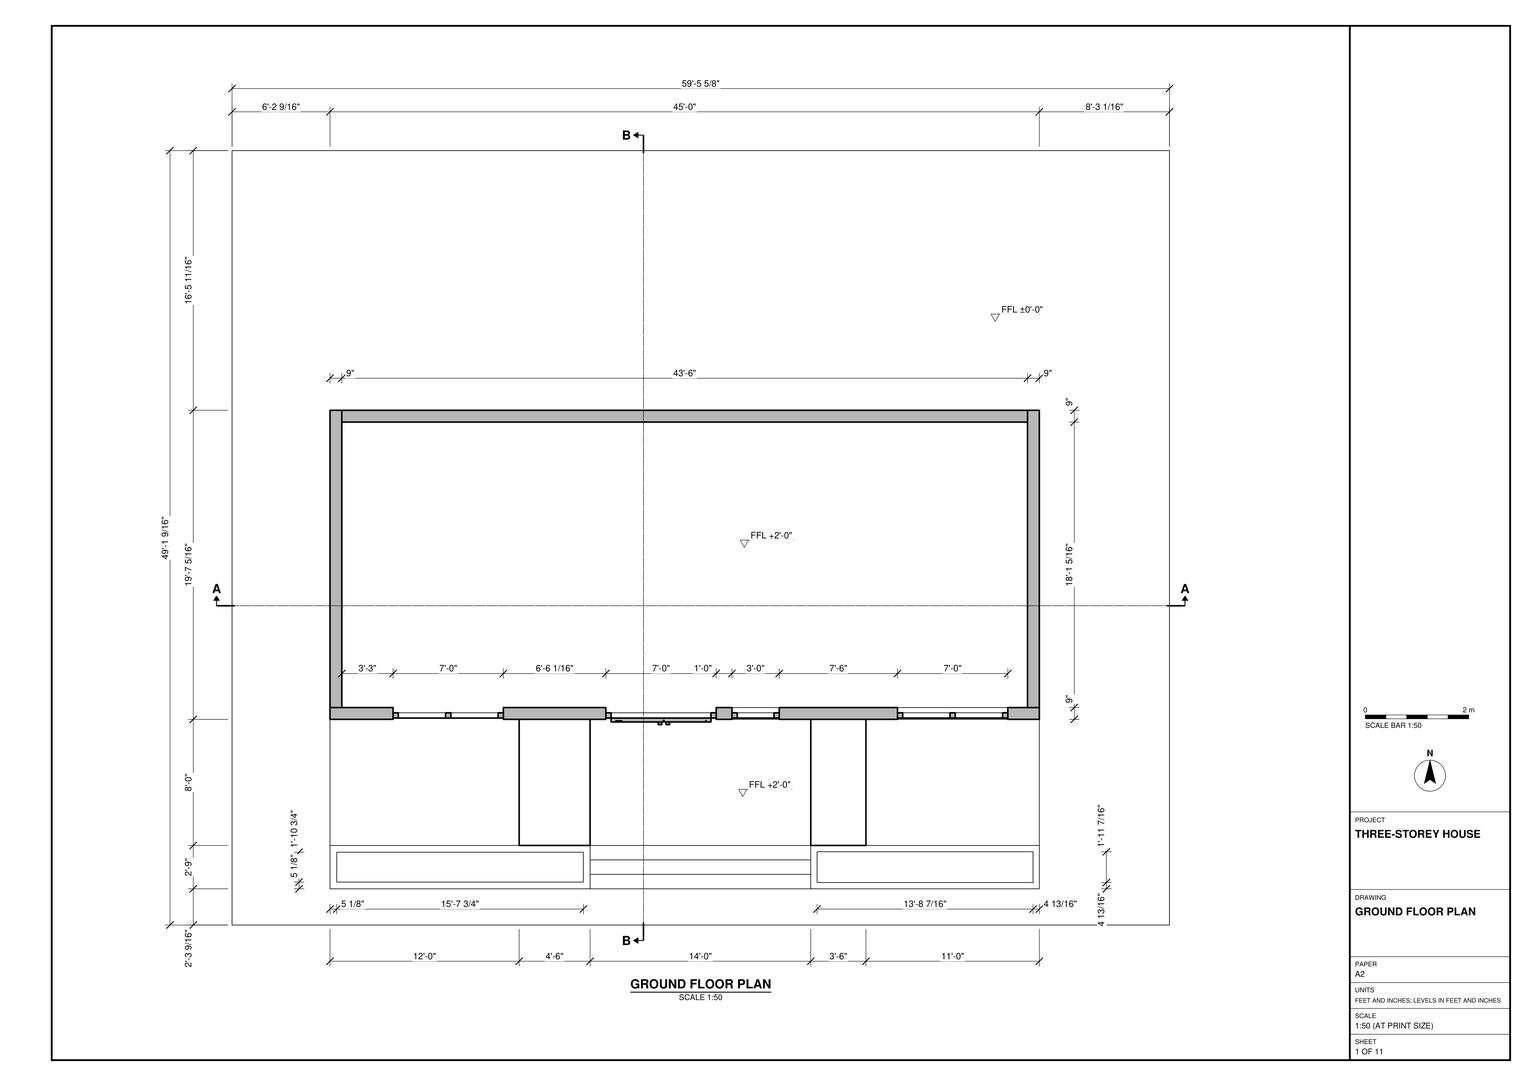
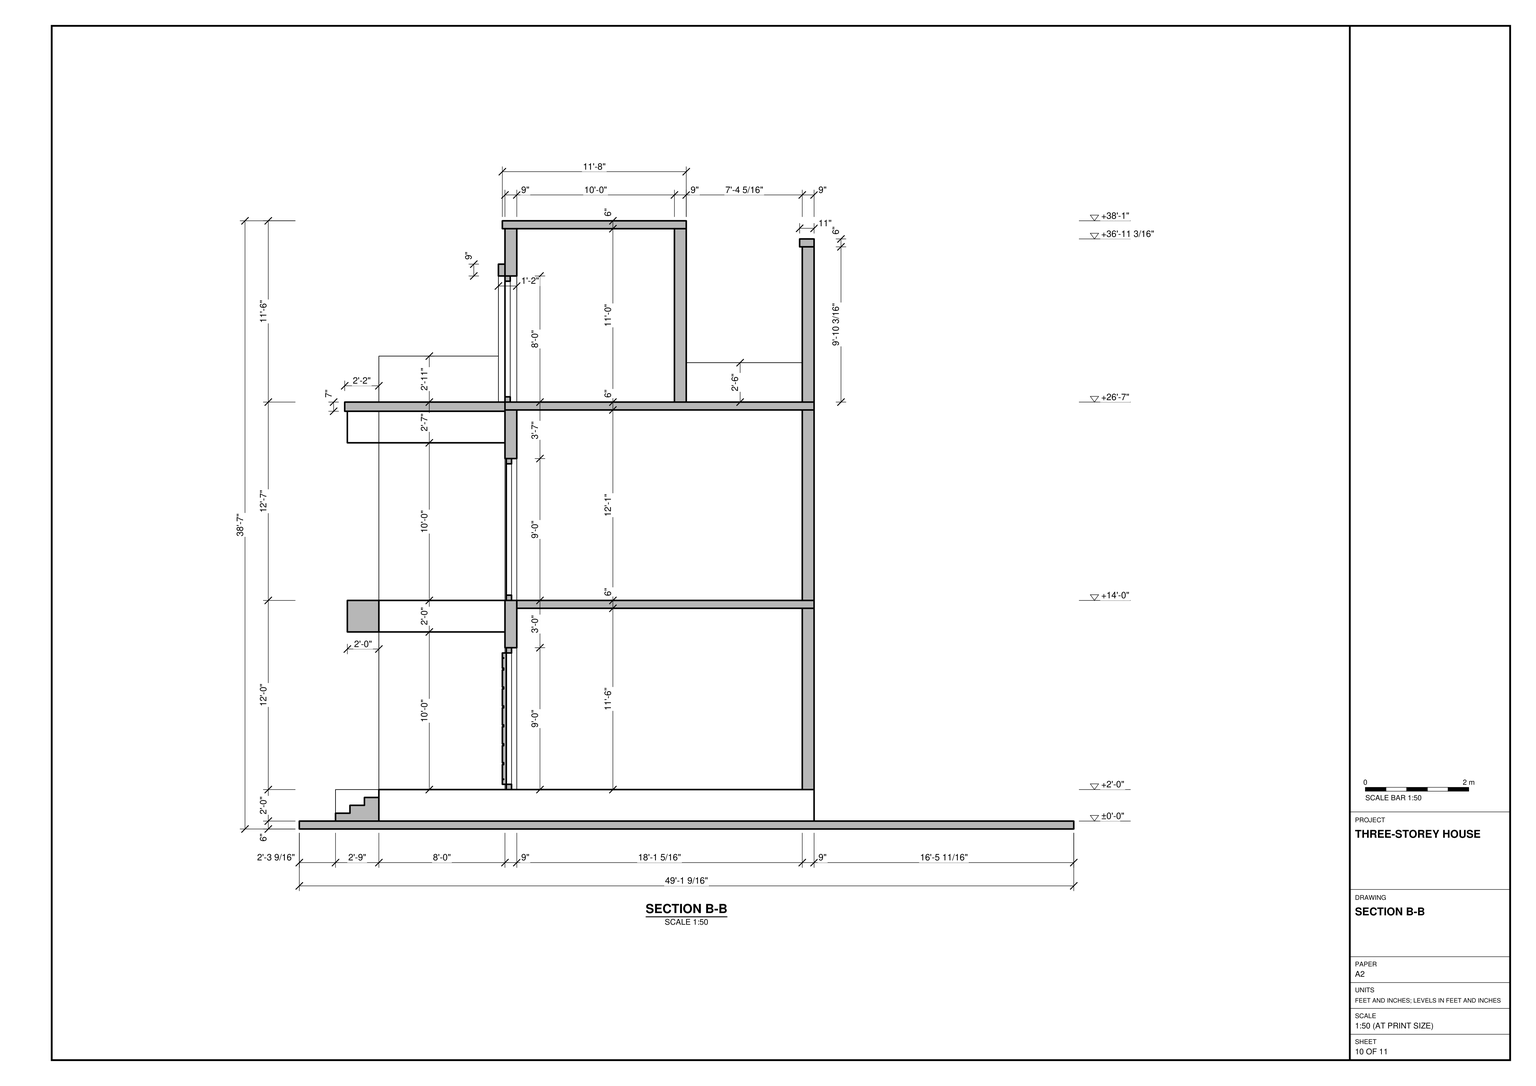
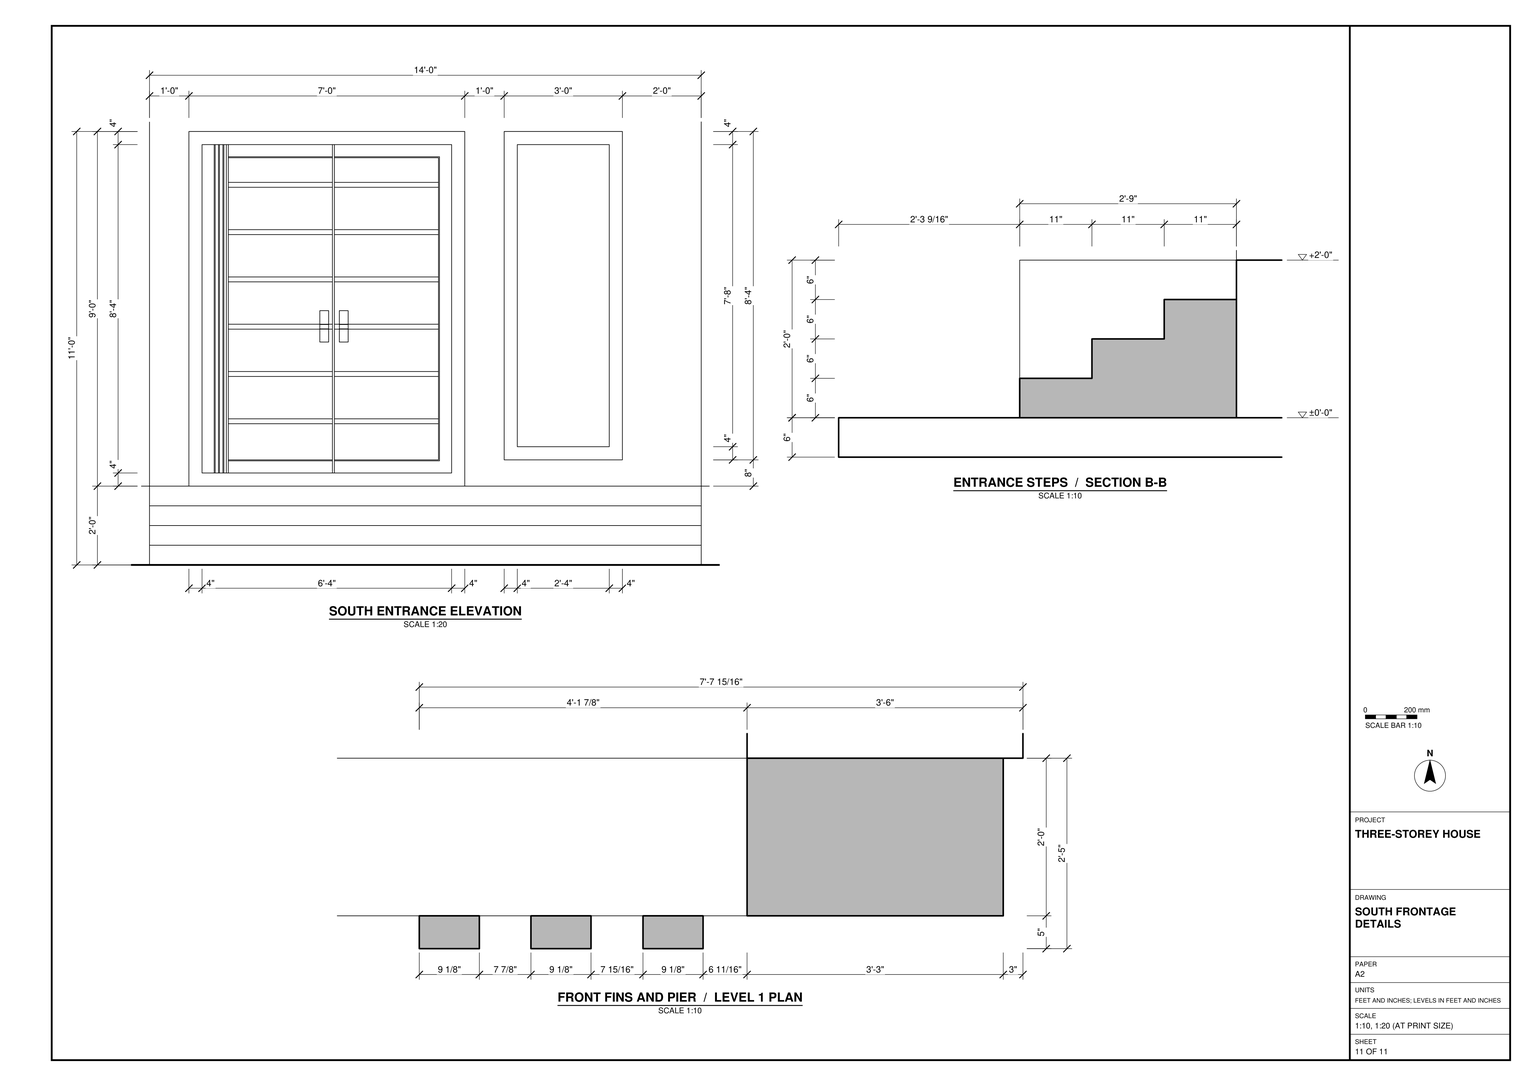
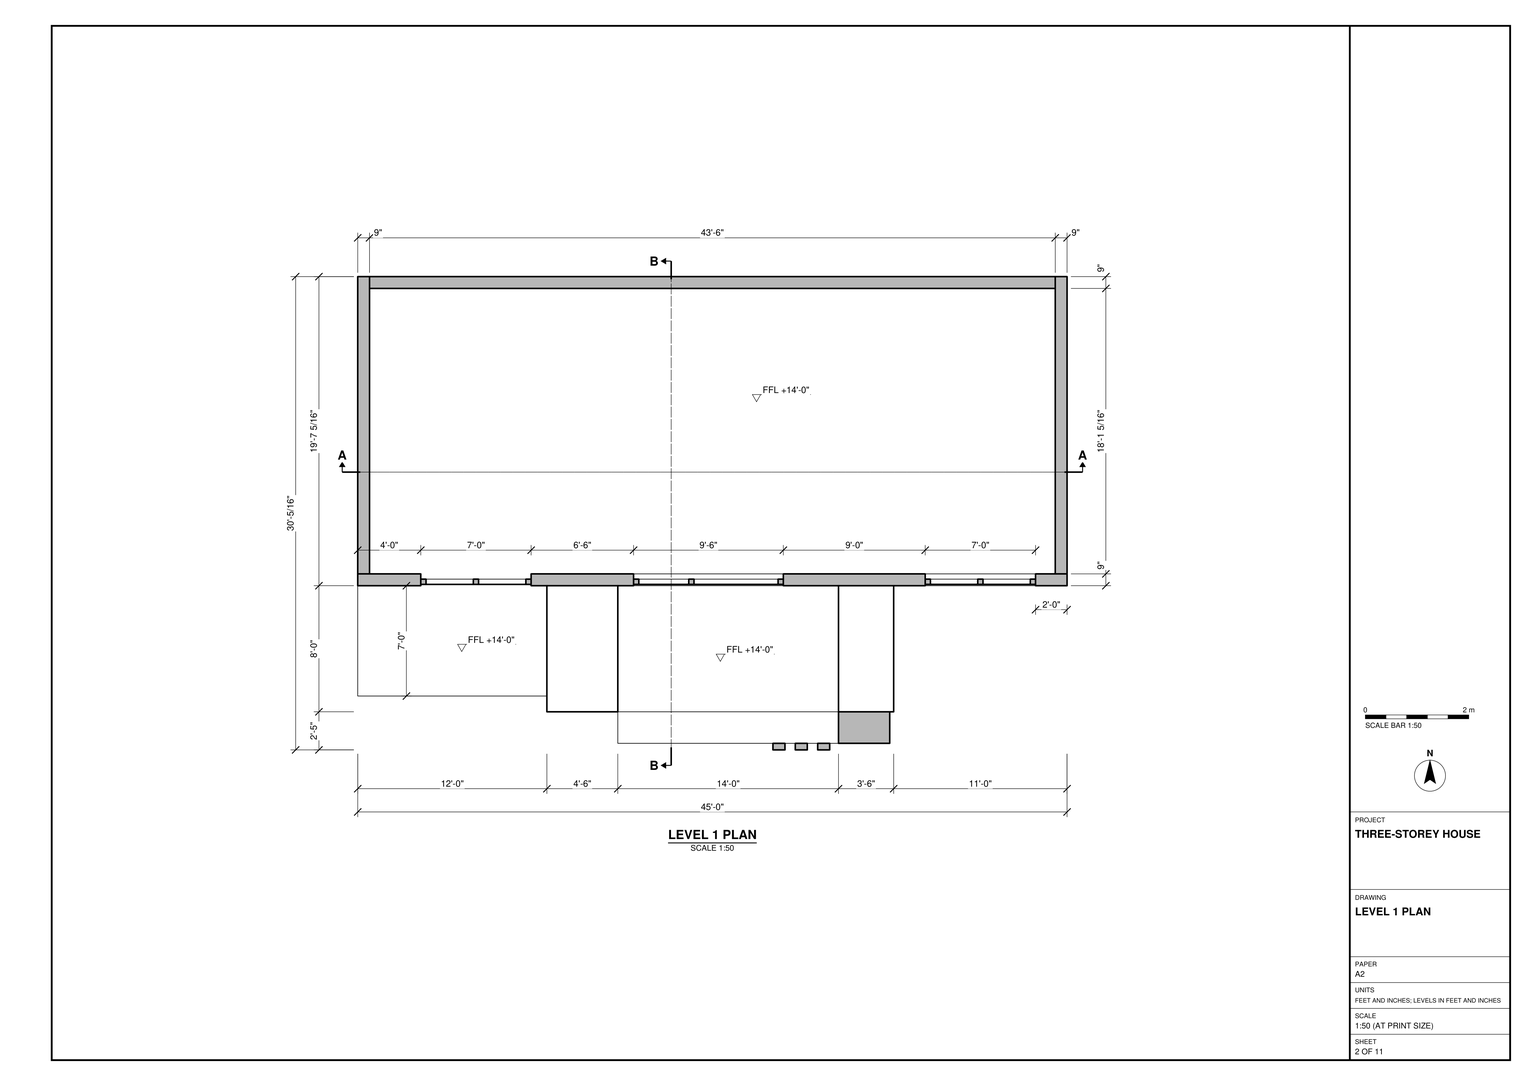
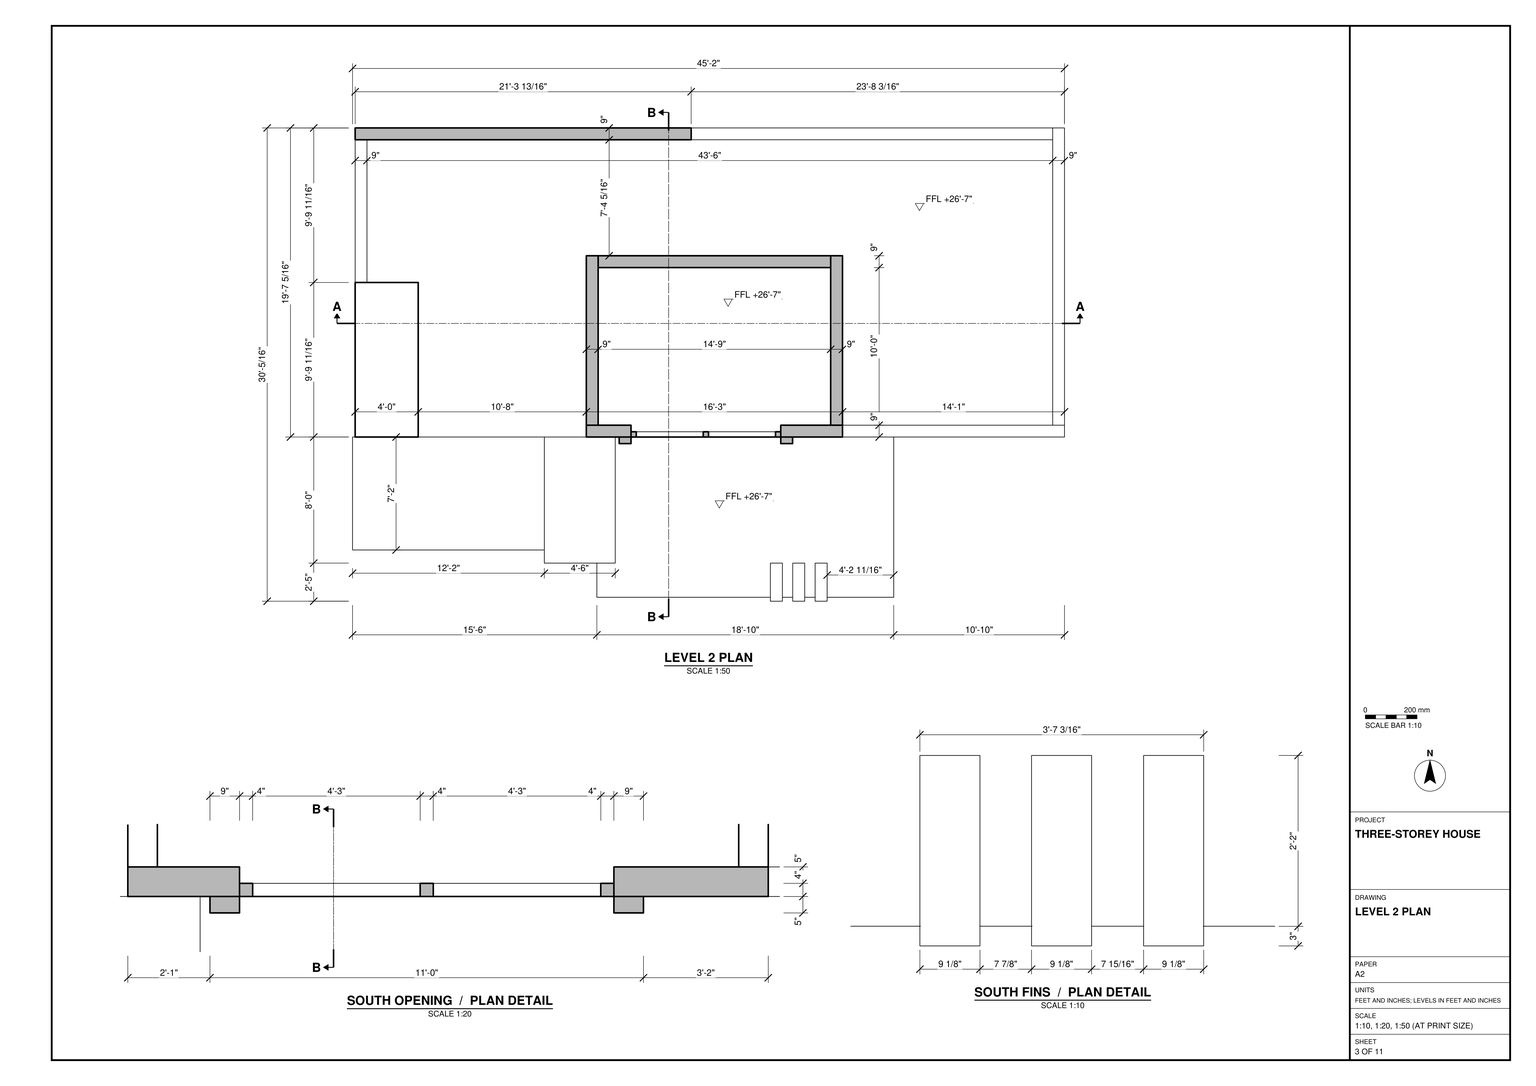
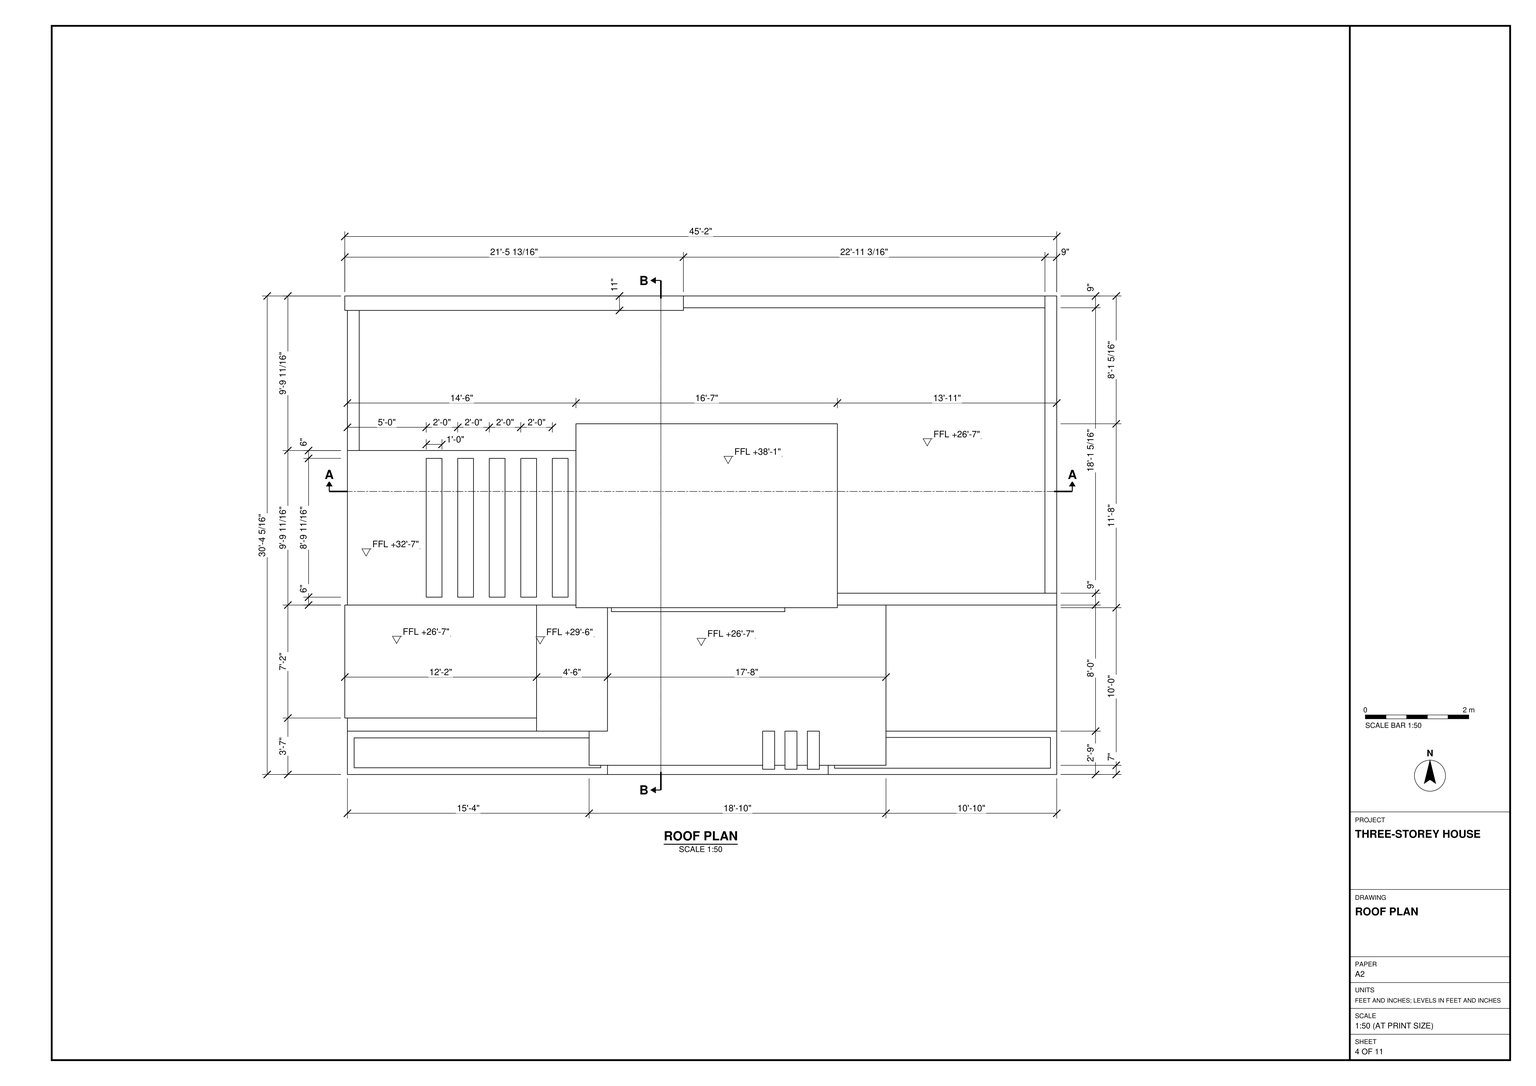
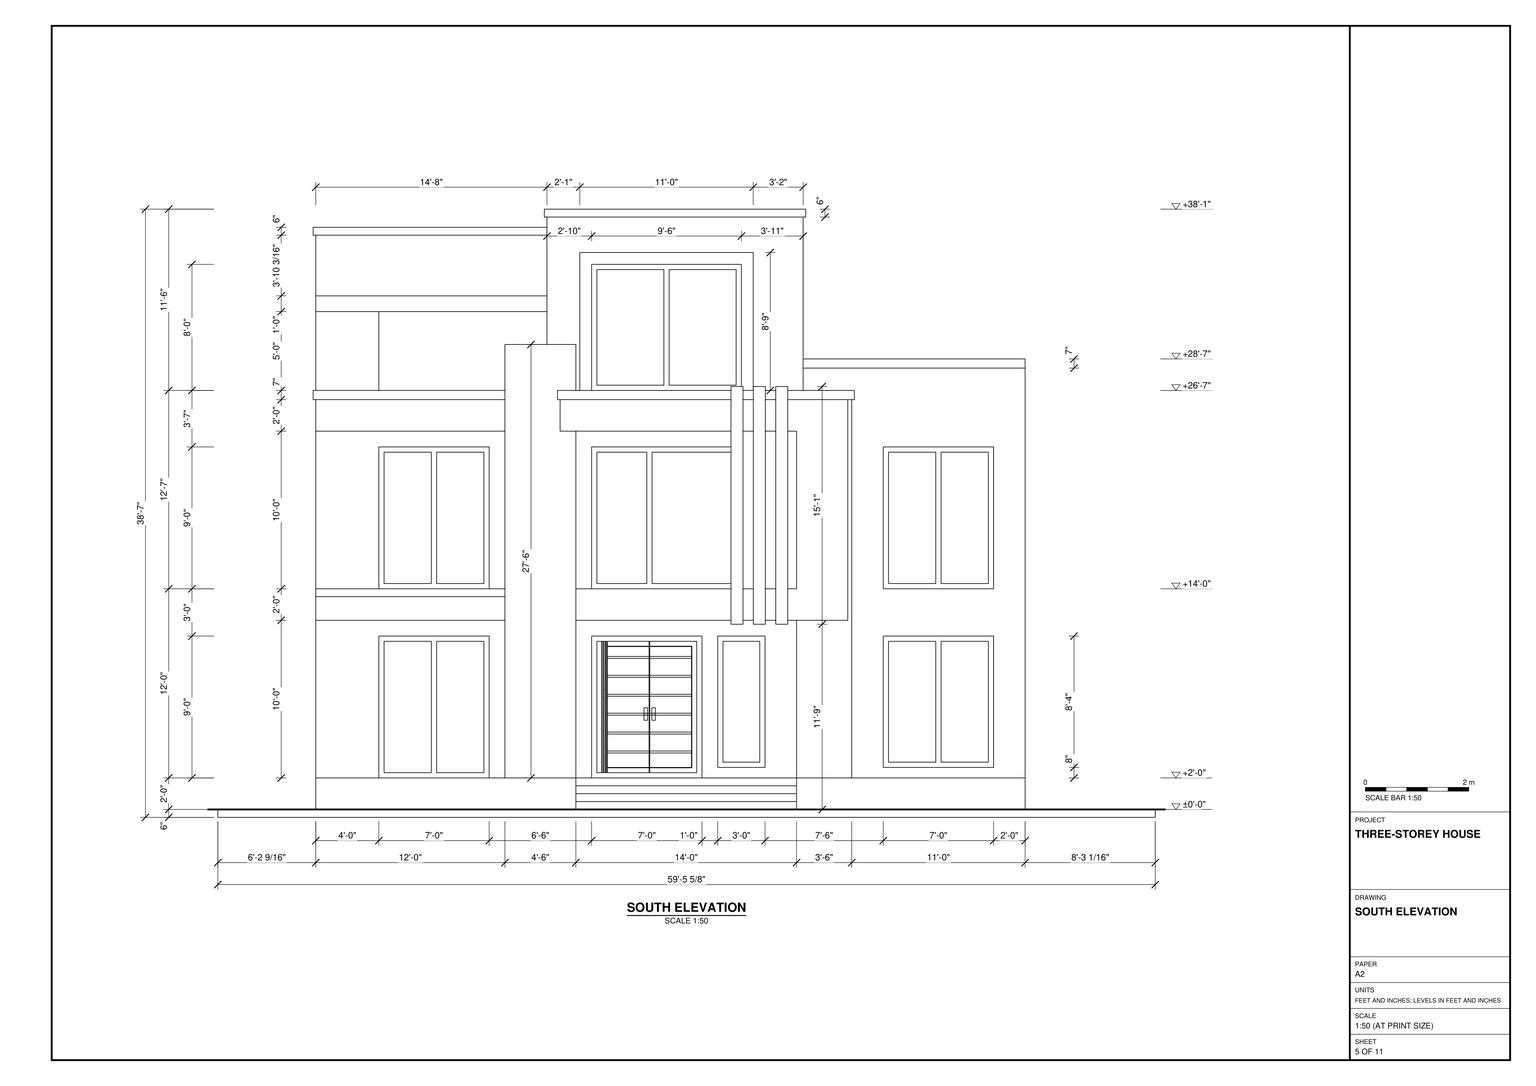
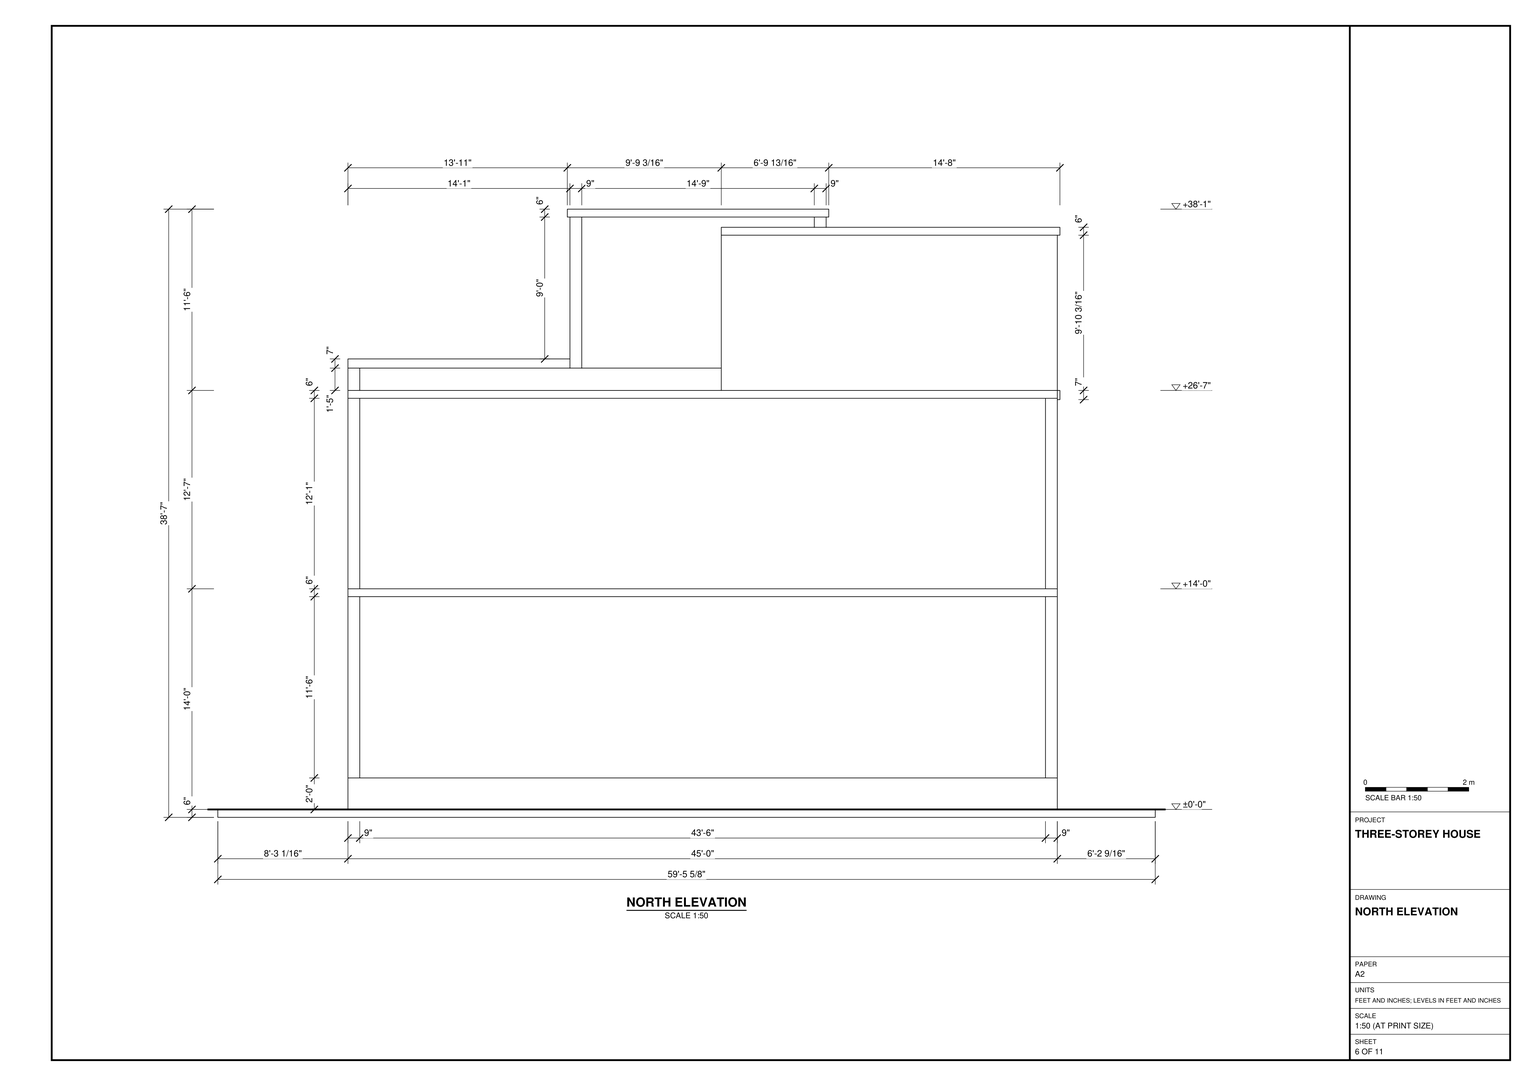
Build the three-storey house and its rectangular site base in SketchUp from task_files/diagram_01.pdf. Work in feet and inches. Including the base, the model must measure 59'-5 5/8" along x, 49'-1 9/16" along y and 38'-7" along z. Use the site surface as the ±0'-0" datum. Set the raised entrance and ground floor at +2'-0" and the upper floors at +14'-0" and +26'-7".

Lay out the shell using the setbacks on the ground floor plan. Follow the plans and sections for wall thicknesses, slab edges, door and window openings, and the flat roof. On the south side, model the steps up to the entrance platform, the double door with its adjacent narrow panel, and the windows to either side of the entrance bay. Use the frontage details to place the fins relative to the pier. Follow section B-B for the projecting floor edges and for the shallower top-floor enclosure and tall wall behind it. Include built-in joinery and main furniture where shown, and leave areas drawn open unobstructed.

Keep walls, slabs and roof elements in separate groups or components. Do the same for each furniture or joinery piece, and use components for repeated parts. Decor and loose items may be any suitable library components. Save one SketchUp model as output_files/three_storey_house_with_a_raised_south_entrance.skp.

# SketchUp Ruby script. Lengths in inches.
U = 1.inch
M = Sketchup.active_model
def pt(a) = Geom::Point3d.new(a.map { |v| v * U })
def face(e, loops, mat)
  f = e.add_face(loops[0].map { |a| pt(a) })
  loops[1..].each { |l| e.add_face(l.map { |a| pt(a) }).erase! }
  f.material = f.back_material = mat if mat
  f
end
# faces: each face lists its corners as indices into pts; further lists are holes
def faces(e, pts, list, mat = nil) = list.each { |f| face(e, (f[0].is_a?(Array) ? f : [f]).map { |l| l.map { |i| pts[i] } }, mat) }
# xy, xz, yz: faces in a plane at the given z, y or x. An outline is a flat list of corners, or four numbers for a rectangle; further outlines are holes
def ring(l) = l.size == 4 ? [[l[0], l[1]], [l[2], l[1]], [l[2], l[3]], [l[0], l[3]]] : l.each_slice(2).to_a
def flat(e, list, mat, &to3) = list.each { |f| face(e, (f[0].is_a?(Array) ? f : [f]).map { |l| ring(l).map { |u, v| to3.(u, v) } }, mat) }
def xy(e, z, list, mat = nil) = flat(e, list, mat) { |x, y| [x, y, z] }
def xz(e, y, list, mat = nil) = flat(e, list, mat) { |x, z| [x, y, z] }
def yz(e, x, list, mat = nil) = flat(e, list, mat) { |y, z| [x, y, z] }
def lines(e, pts, list) = list.each { |a, b| e.add_line(pt(pts[a]), pt(pts[b])) }
# prism: a flat outline (further loops are holes) pulled along v
def prism(e, loops, v, mat = nil)
  f = face(e, loops, mat); d = Geom::Vector3d.new(v.map { |x| x * U })
  f.pushpull(f.normal.samedirection?(d) ? d.length : -d.length)
end
def box(e, o, s, mat = nil) = prism(e, [[o, [o[0] + s[0], o[1], o[2]], [o[0] + s[0], o[1] + s[1], o[2]], [o[0], o[1] + s[1], o[2]]]], [0, 0, s[2]], mat)
def at(x, y, z, deg = 0) = Geom::Transformation.translation(pt([x, y, z])) * Geom::Transformation.rotation(ORIGIN, Z_AXIS, deg.degrees)
def axes(o, x, y, z) = Geom::Transformation.new([*x, 0, *y, 0, *z, 0, *pt(o).to_a, 1])
def part(name) = M.definitions.add(name)
# library, detail: a bought-in or finely detailed component or shape, given as its bounding box
def library(name, o, s) = part(name).tap { |d| box(d.entities, o, s) }
def detail(e, o, s) = box(e.add_group.entities, o, s)
def put(e, d, t, mat = nil) = e.add_instance(d, t).tap { |i| i.material = mat if mat }
def group(e, t, mat = nil) = e.add_group.tap { |g| g.transformation = t; g.material = mat if mat }.entities
root = M.entities
M.materials.add("[Aluminum]").color = [179, 179, 179]
M.materials.add("[Color M06]").color = [86, 86, 86]
M.materials.add("[Color M07]").color = [58, 58, 58]
M.materials.add("[Field Rectangle Tile]").color = [196, 189, 179]
M.materials.add("[Grass Dark Green]").color = [106, 157, 55]
M.materials.add("[Translucent Glass Gray]").color = [128, 128, 128]
M.materials["[Translucent Glass Gray]"].alpha = 0.5
M.materials.add("[Wood Floor Dark]").color = [153, 94, 42]
M.materials.add("[Wood Veneer 01]").color = [120, 70, 37]
c1 = part("Group\#10")
prism(c1.entities,[[[2.6875,2,0],[2.6875,2,9.5625],[2.6875,0,9.5625],[2.6875,0,5.43],[2.6875,0.3,5.43],[2.6875,0.3,5.34],[2.6875,0,5.34],[2.6875,0,4.01],[2.6875,0.3,4.01],[2.6875,0.3,3.93],[2.6875,0,3.93],[2.6875,0,0]]],[-2.6875,0,0])
xz(root,157.56,[[126.57,34,162.57,134]],"[Translucent Glass Gray]")
g1 = group(root,at(0,-75.0625,0))
box(g1,[0,75.0625,0],[713.625,589.5625,6])
g2 = group(root,at(132.17,60.56,6))
box(g2,[-57.6,0,0],[540,331.3125,24])
g3 = group(root,at(132.17,156.56,30))
prism(g3,[[[-9.6,9,0],[-57.6,9,0],[-57.6,9,138],[86.4,9,138],[86.4,9,144],[74.4,9,144],[74.4,9,252],[-9.6,9,252],[-9.6,9,144],[-57.6,9,144],[-57.6,9,289],[352.4,9,289],[352.4,9,295],[313.4,9,295],[313.4,9,312],[482.4,9,312],[482.4,9,0],[236.4,9,0],[236.4,9,108],[152.4,9,108],[152.4,9,0],[74.4,9,0],[74.4,9,108],[-9.6,9,108]],[[152.4,9,252],[152.4,9,144],[266.4,9,144],[266.4,9,252]],[[374.4,9,144],[458.4,9,144],[458.4,9,252],[374.4,9,252]],[[458.4,9,108],[374.4,9,108],[374.4,9,8],[458.4,9,8]],[[248.4,9,108],[248.4,9,8],[284.4,9,8],[284.4,9,108]]],[0,-9,0])
g4 = group(root,at(506.57,157.56,38),"[Color M07]")
prism(g4,[[[84,4,100],[84,4,0],[0,4,0],[0,4,100]],[[40,4,4],[40,4,96],[4,4,96],[4,4,4]],[[80,4,96],[44,4,96],[44,4,4],[80,4,4]]],[0,-4,0])
g5 = group(root,at(380.57,157.56,38),"[Color M07]")
prism(g5,[[[36,4,100],[36,4,0],[0,4,0],[0,4,100]],[[4,4,96],[4,4,4],[32,4,4],[32,4,96]]],[0,-4,0])
g6 = group(root,at(284.57,157.56,30),"[Wood Veneer 01]")
prism(g6,[[[0,4,0],[0,4,108],[84,4,108],[84,4,0]],[[4,4,4],[80,4,4],[80,4,104],[4,4,104]]],[0,-4,0])
g7 = group(root,at(440.57,60.56,30),"[Field Rectangle Tile]")
box(g7,[0,0,0],[42,96,293])
g8 = group(root,at(288.57,155.56,34),"[Wood Veneer 01]")
xy(g8,0,[[0,-1,0,2,76,2,76,-1,40.3,-1,40.3,0.3,39.7,0.3,39.7,-1,8,-1,8,0,7.4,0,7.4,-1,6.65,-1,6.65,0,6.35,0,6.35,-1,5.3,-1,5.3,0,5,0,5,-1,4,-1,4,0,3.7,0,3.7,-1]])
xy(g8,3.7,[[8,-1,39.7,0],[40.3,-1,72.3,0]])
xy(g8,4,[[8,-1,39.7,0],[40.3,-1,72,0]])
xy(g8,15,[[8,-1,39.7,0],[40.3,-1,72,0]])
xy(g8,16.5,[[8,-1,39.7,0],[40.3,-1,72,0]])
xy(g8,29.4,[[8,-1,39.7,0],[40.3,-1,72,0]])
xy(g8,30.9,[[8,-1,39.7,0],[40.3,-1,72,0]])
xy(g8,43.8,[[8,-1,39.7,0],[40.3,-1,72,0]])
xy(g8,45.3,[[8,-1,39.7,0],[40.3,-1,72,0]])
xy(g8,58.2,[[8,-1,39.7,0],[40.3,-1,72,0]])
xy(g8,59.7,[[8,-1,39.7,0],[40.3,-1,72,0]])
xy(g8,72.6,[[8,-1,39.7,0],[40.3,-1,72,0]])
xy(g8,74.1,[[8,-1,39.7,0],[40.3,-1,72,0]])
xy(g8,87,[[8,-1,39.7,0],[40.3,-1,72,0]])
xy(g8,88.5,[[8,-1,39.7,0],[40.3,-1,72,0]])
xy(g8,96,[[8,-1,39.7,0],[40.3,-1,72,0]])
xy(g8,96.3,[[8,-1,39.7,0],[40.3,-1,72.3,0]])
xy(g8,100,[[0,-1,3.7,-1,3.7,0,4,0,4,-1,5,-1,5,0,5.3,0,5.3,-1,6.35,-1,6.35,0,6.65,0,6.65,-1,7.4,-1,7.4,0,8,0,8,-1,39.7,-1,39.7,0.3,40.3,0.3,40.3,-1,76,-1,76,2,0,2]])
xz(g8,-1,[[0,0,3.7,100],[4,0,5,100],[5.3,0,6.35,100],[6.65,0,7.4,100],[8,0,39.7,3.7],
  [40.3,0,76,0,76,100,40.3,100,40.3,96.3,72.3,96.3,72.3,3.7,40.3,3.7],[8,4,39.7,15],[40.3,4,72,15],[8,16.5,39.7,29.4],[40.3,16.5,72,29.4],
  [8,30.9,39.7,43.8],[40.3,30.9,72,43.8],[8,45.3,39.7,58.2],[40.3,45.3,72,58.2],[8,59.7,39.7,72.6],
  [40.3,59.7,72,72.6],[8,74.1,39.7,87],[40.3,74.1,72,87],[8,88.5,39.7,96],[40.3,88.5,72,96],
  [8,96.3,39.7,100]])
xz(g8,0,[[3.7,0,4,100],[5,0,5.3,100],[6.35,0,6.65,100],[7.4,0,8,100],[8,3.7,39.7,4],
  [40.3,3.7,72.3,3.7,72.3,96.3,40.3,96.3,40.3,96,72,96,72,4,40.3,4],[8,15,39.7,16.5],[40.3,15,72,16.5],[8,29.4,39.7,30.9],[40.3,29.4,72,30.9],
  [8,43.8,39.7,45.3],[40.3,43.8,72,45.3],[8,58.2,39.7,59.7],[40.3,58.2,72,59.7],[8,72.6,39.7,74.1],
  [40.3,72.6,72,74.1],[8,87,39.7,88.5],[40.3,87,72,88.5],[8,96,39.7,96.3]])
xz(g8,0.3,[[39.7,0,40.3,100]])
xz(g8,2,[[0,0,76,100]])
yz(g8,0,[[-1,0,2,100]])
yz(g8,3.7,[[-1,0,0,100]])
yz(g8,4,[[-1,0,0,100]])
yz(g8,5,[[-1,0,0,100]])
yz(g8,5.3,[[-1,0,0,100]])
yz(g8,6.35,[[-1,0,0,100]])
yz(g8,6.65,[[-1,0,0,100]])
yz(g8,7.4,[[-1,0,0,100]])
yz(g8,8,[[-1,0,0,3.7],[-1,4,0,15],[-1,16.5,0,29.4],[-1,30.9,0,43.8],[-1,45.3,0,58.2],
  [-1,59.7,0,72.6],[-1,74.1,0,87],[-1,88.5,0,96],[-1,96.3,0,100]])
yz(g8,39.7,[[-1,0,0.3,3.7],[0,3.7,0.3,4],[-1,4,0.3,15],[0,15,0.3,16.5],[-1,16.5,0.3,29.4],
  [0,29.4,0.3,30.9],[-1,30.9,0.3,43.8],[0,43.8,0.3,45.3],[-1,45.3,0.3,58.2],[0,58.2,0.3,59.7],
  [-1,59.7,0.3,72.6],[0,72.6,0.3,74.1],[-1,74.1,0.3,87],[0,87,0.3,88.5],[-1,88.5,0.3,96],
  [0,96,0.3,96.3],[-1,96.3,0.3,100]])
yz(g8,40.3,[[-1,0,0.3,3.7],[0,3.7,0.3,4],[-1,4,0.3,15],[0,15,0.3,16.5],[-1,16.5,0.3,29.4],
  [0,29.4,0.3,30.9],[-1,30.9,0.3,43.8],[0,43.8,0.3,45.3],[-1,45.3,0.3,58.2],[0,58.2,0.3,59.7],
  [-1,59.7,0.3,72.6],[0,72.6,0.3,74.1],[-1,74.1,0.3,87],[0,87,0.3,88.5],[-1,88.5,0.3,96],
  [0,96,0.3,96.3],[-1,96.3,0.3,100]])
yz(g8,72,[[-1,4,0,15],[-1,16.5,0,29.4],[-1,30.9,0,43.8],[-1,45.3,0,58.2],[-1,59.7,0,72.6],
  [-1,74.1,0,87],[-1,88.5,0,96]])
yz(g8,72.3,[[-1,3.7,0,96.3]])
yz(g8,76,[[-1,0,2,100]])
put(root,c1,at(330.37,152.56,73.875),"[Aluminum]")
put(root,c1,at(324.43,152.56,73.875),"[Aluminum]")
g9 = group(root,at(122.57,157.56,30),"[Color M07]")
prism(g9,[[[84,0,108],[0,0,108],[0,0,0],[84,0,0]],[[40,0,104],[40,0,4],[4,0,4],[4,0,104]],[[44,0,104],[80,0,104],[80,0,4],[44,0,4]]],[0,4,0])
g10 = group(root,at(166.57,157.56,34),"[Translucent Glass Gray]")
xz(g10,0,[[0,0,36,100]])
g11 = group(root,at(384.57,157.56,42),"[Translucent Glass Gray]")
xz(g11,0,[[0,0,28,92]])
g12 = group(root,at(550.57,157.56,42),"[Translucent Glass Gray]")
xz(g12,0,[[0,0,36,92]])
g13 = group(root,at(510.57,157.56,42),"[Translucent Glass Gray]")
xz(g13,0,[[0,0,36,92]])
g14 = group(root,at(218.57,96.56,30),"[Wood Floor Dark]")
box(g14,[0,-36,0],[54,96,330])
g15 = group(root,at(74.57,165.56,30))
box(g15,[0,0,0],[9,226.3125,138])
g16 = group(root,at(605.57,165.56,30))
box(g16,[0,0,0],[9,226.3125,138])
g17 = group(root,at(83.57,382.88,30))
box(g17,[0,0,0],[522,9,138])
g18 = group(root,at(74.57,156.56,150))
box(g18,[0,-84,0],[144,84,18])
g19 = group(root,at(74.57,165.56,168))
prism(g19,[[[0,226.3125,0],[540,226.3125,0],[540,0,0],[144,0,0],[144,-93,0],[0,-93,0]]],[0,0,6])
g20 = group(root,at(506.57,157.56,174))
xy(g20,0,[[0,0,84,4]],"[Color M06]")
xy(g20,4,[[4,0,40,4],[44,0,80,4]],"[Color M06]")
xy(g20,104,[[4,0,40,4],[44,0,80,4]],"[Color M06]")
xy(g20,108,[[0,0,84,4]],"[Color M06]")
xz(g20,0,[[[0,0,84,108],[4,4,40,104],[44,4,80,104]]],"[Color M07]")
xz(g20,4,[[[0,0,84,108],[4,4,40,104],[44,4,80,104]]],"[Color M06]")
yz(g20,0,[[0,0,4,108]],"[Color M06]")
yz(g20,4,[[0,4,4,104]],"[Color M06]")
yz(g20,40,[[0,4,4,104]],"[Color M06]")
yz(g20,44,[[0,4,4,104]],"[Color M06]")
yz(g20,80,[[0,4,4,104]],"[Color M06]")
yz(g20,84,[[0,0,4,108]],"[Color M06]")
g21 = group(root,at(550.57,157.56,178),"[Translucent Glass Gray]")
xz(g21,0,[[0,0,36,100]])
g22 = group(root,at(510.57,157.56,178),"[Translucent Glass Gray]")
xz(g22,0,[[0,0,36,100]])
g23 = group(root,at(272.57,72.56,150))
box(g23,[0,-12,0],[168,96,24])
g24 = group(root,at(284.57,157.56,174),"[Color M07]")
prism(g24,[[[114,0,108],[0,0,108],[0,0,0],[114,0,0]],[[46,0,104],[110,0,104],[110,0,4],[46,0,4]],[[42,0,104],[42,0,4],[4,0,4],[4,0,104]]],[0,4,0])
g25 = group(root,at(330.57,157.56,178),"[Translucent Glass Gray]")
xz(g25,0,[[0,0,64,100]])
g26 = group(root,at(288.57,157.56,178),"[Translucent Glass Gray]")
xz(g26,0,[[0,0,38,100]])
g27 = group(root,at(122.57,158.56,174),"[Color M07]")
prism(g27,[[[84,3,108],[84,3,0],[0,3,0],[0,3,108]],[[44,3,104],[44,3,4],[80,3,4],[80,3,104]],[[4,3,4],[40,3,4],[40,3,104],[4,3,104]]],[0,-4,0])
g28 = group(root,at(166.57,157.56,178),"[Translucent Glass Gray]")
xz(g28,0,[[0,0,36,100]])
g29 = group(root,at(126.57,157.56,178),"[Translucent Glass Gray]")
xz(g29,0,[[0,0,36,100]])
g30 = group(root,at(74.57,165.56,174))
box(g30,[0,0,0],[9,226.3125,145])
g31 = group(root,at(605.57,165.56,174))
box(g31,[0,0,0],[9,226.3125,145])
g32 = group(root,at(83.57,382.88,174))
box(g32,[0,0,0],[522,9,145])
g33 = group(root,at(272.57,36.56,150))
xy(g33,0,[[0,0,207,24]])
xy(g33,24,[[0,0,168,24]])
xy(g33,144,[[-12,0,-12,36,-198,36,-198,120,168,120,168,0],[168,24,207,120]])
xy(g33,168,[[-12,0,207,0,207,120,-198,120,-198,36,-12,36]])
xz(g33,0,[[0,0,207,0,207,168,-12,168,-12,144,168,144,168,24,0,24]])
xz(g33,24,[[0,0,0,24,168,24,168,144,207,144,207,0]])
xz(g33,36,[[-198,144,-12,168]])
xz(g33,120,[[-198,144,207,168]])
yz(g33,-198,[[36,144,120,168]])
yz(g33,-12,[[0,144,36,168]])
yz(g33,0,[[0,0,24,24]])
yz(g33,168,[[0,24,24,144]])
yz(g33,207,[[0,0,24,0,24,144,120,144,120,168,0,168]])
g34 = group(root,at(74.57,165.56,319))
prism(g34,[[[540,226.3125,0],[540,0,0],[410,0,0],[410,-9,0],[0,-9,0],[0,226.3125,0]]],[0,0,6])
g35 = group(root,at(72.57,34.56,294),"[Color M06]")
xy(g35,24,[[186,0,186,36,188,36,188,122,412,122,412,0],[0,36,188,122]])
xy(g35,31,[[186,0,412,0,412,122,0,122,0,36,186,36]])
xz(g35,0,[[186,24,412,31]])
xz(g35,36,[[0,24,186,31]])
xz(g35,122,[[0,24,188,31],[188,24,410,31],[410,24,412,31]])
yz(g35,0,[[36,24,122,31]])
yz(g35,186,[[0,24,36,31]])
yz(g35,412,[[0,24,122,31]])
p = [[188,36,24],[188,36,30],[410,122,24],[410,122,0],[410,131,0]]
lines(g35,p,[[0,1],[2,3],[3,4]])
g36 = group(root,at(74.57,156.56,325))
box(g36,[0,0,0],[48,117.66,60])
g37 = group(root,at(74.57,156.56,385),"[Color M06]")
prism(g37,[[[175.98,117.66,0],[175.98,0,0],[0,0,0],[0,117.66,0]],[[72,6,0],[72,111.66,0],[60,111.66,0],[60,6,0]],[[96,111.66,0],[84,111.66,0],[84,6,0],[96,6,0]],[[108,6,0],[120,6,0],[120,111.66,0],[108,111.66,0]],[[132,6,0],[144,6,0],[144,111.66,0],[132,111.66,0]],[[168,111.66,0],[156,111.66,0],[156,6,0],[168,6,0]]],[0,0,12])
g38 = group(root,at(250.55,156.56,325))
prism(g38,[[[195.02,9,0],[148.02,9,0],[148.02,9,96],[34.02,9,96],[34.02,9,0],[0,9,0],[0,9,132],[195.02,9,132]]],[0,-9,0])
g39 = group(root,at(275.57,151.56,325))
prism(g39,[[[132,5,0],[123,5,0],[123,5,96],[9,5,96],[9,5,0],[0,5,0],[0,5,105],[132,5,105]]],[0,-5,0])
p = [[9,5,0],[123,5,0]]
lines(g39,p,[[0,1]])
g40 = group(root,at(284.57,156.56,325),"[Color M07]")
prism(g40,[[[0,4,0],[0,4,96],[114,4,96],[114,4,0]],[[55,4,4],[55,4,92],[4,4,92],[4,4,4]],[[110,4,92],[59,4,92],[59,4,4],[110,4,4]]],[0,-4,0])
g41 = group(root,at(343.57,156.56,329),"[Translucent Glass Gray]")
xz(g41,0,[[0,0,51,88]])
g42 = group(root,at(288.57,156.56,329),"[Translucent Glass Gray]")
xz(g42,0,[[0,0,51,88]])
g43 = group(root,at(250.55,156.56,457),"[Color M06]")
box(g43,[-2,-2,0],[199.02,140,6])
g44 = group(root,at(250.55,165.56,325))
box(g44,[0,0,0],[9,129,132])
g45 = group(root,at(436.57,165.56,325))
box(g45,[0,0,0],[9,129,132])
g46 = group(root,at(259.55,285.56,325))
box(g46,[0,0,0],[177.02,9,132])
g47 = group(root,at(484.57,156.56,342),"[Color M06]")
box(g47,[-39,0,0],[169,9,7])
g48 = group(root,at(420.72,31.56,147),"[Color M06]")
prism(g48,[[[13.15,5,3],[13.15,5,178],[13.15,29,178],[13.15,29,181],[13.15,0,181],[13.15,0,0],[13.15,29,0],[13.15,29,3]]],[-9.15,0,0])
g49 = group(root,at(403.66,31.56,147),"[Color M06]")
prism(g49,[[[13.15,5,3],[13.15,5,178],[13.15,29,178],[13.15,29,181],[13.15,0,181],[13.15,0,0],[13.15,29,0],[13.15,29,3]]],[-9.15,0,0])
g50 = group(root,at(386.66,31.56,147),"[Color M06]")
prism(g50,[[[13.15,5,3],[13.15,5,178],[13.15,29,178],[13.15,29,181],[13.15,0,181],[13.15,0,0],[13.15,29,0],[13.15,29,3]]],[-9.15,0,0])
g51 = group(root,at(74.57,382.88,325))
box(g51,[0,0,0],[255.8,9,118.1875])
g52 = group(root,at(72.57,380.88,443.1875),"[Color M06]")
box(g52,[0,0,0],[257.8,11,6])
g53 = group(root,at(272.57,27.56,6))
xy(g53,0,[[0,0,168,33],[168,0,342,33]])
xy(g53,6,[[0,0,168,11]])
xy(g53,12,[[0,11,168,22]])
xy(g53,18,[[0,22,168,33]])
xy(g53,23,[[172.79,4.79,337.21,28.21]],"[Grass Dark Green]")
xy(g53,24,[[[168,0,342,33],[172.79,4.79,337.21,28.21]]],"[Color M06]")
xz(g53,0,[[0,0,168,6]])
xz(g53,0,[[168,0,342,24]],"[Color M06]")
xz(g53,4.79,[[172.79,23,337.21,24]])
xz(g53,11,[[0,6,168,12]])
xz(g53,22,[[0,12,168,18]])
xz(g53,28.21,[[172.79,23,337.21,24]])
xz(g53,33,[[0,0,168,18],[168,0,342,24]])
yz(g53,0,[[0,0,0,6,11,6,11,12,22,12,22,18,33,18,33,0]])
yz(g53,168,[[0,0,0,6,11,6,11,12,22,12,22,18,33,18,33,0]])
yz(g53,168,[[0,6,0,24,33,24,33,18,22,18,22,12,11,12,11,6]],"[Color M06]")
yz(g53,172.79,[[4.79,23,28.21,24]])
yz(g53,337.21,[[4.79,23,28.21,24]])
yz(g53,342,[[0,0,33,24]],"[Color M06]")
g54 = group(root,at(74.57,27.56,6),"[Grass Dark Green]")
xy(g54,0,[[0,0,198,33]])
xy(g54,22.125,[[5.13,5.13,192.87,27.87]])
xy(g54,24,[[[0,0,198,33],[5.13,5.13,192.87,27.87]]],"[Color M06]")
xz(g54,0,[[0,0,198,24]],"[Color M06]")
xz(g54,5.13,[[5.13,22.125,192.87,24]])
xz(g54,27.87,[[5.13,22.125,192.87,24]])
xz(g54,33,[[0,0,198,24]])
yz(g54,0,[[0,0,33,24]],"[Color M06]")
yz(g54,5.13,[[5.13,22.125,27.87,24]])
yz(g54,192.87,[[5.13,22.125,27.87,24]])
yz(g54,198,[[0,0,33,24]])
g55 = group(root,at(605.57,165.56,325))
box(g55,[0,0,0],[9,226.3125,17])
g56 = group(root,at(330.36,382.88,325))
box(g56,[0,0,0],[275.2,9,17])
g57 = group(root,at(74.57,274.22,325))
box(g57,[0,0,0],[9,108.66,30])
